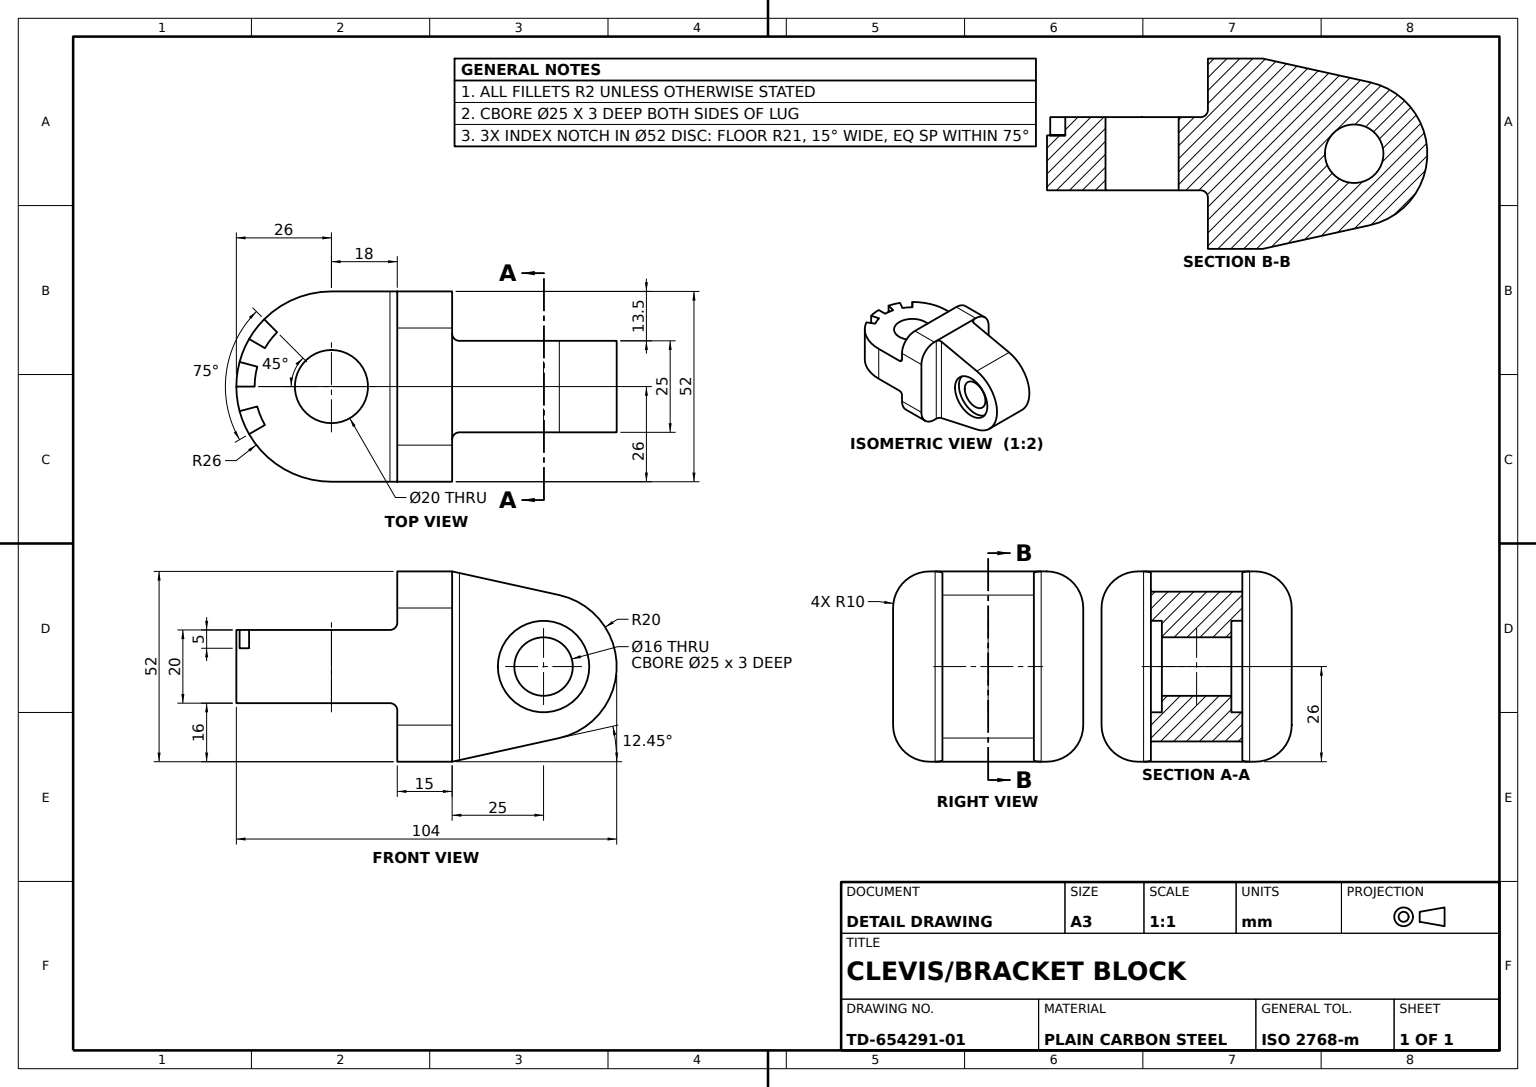
ISO-10303-21;
HEADER;
FILE_DESCRIPTION((''),'2;1');
FILE_NAME('','',(''),(''),'','','');
FILE_SCHEMA(('AUTOMOTIVE_DESIGN'));
ENDSEC;
DATA;
#1=APPLICATION_CONTEXT('');
#2=PRODUCT_CONTEXT('',#1,'mechanical');
#3=PRODUCT('','','',(#2));
#4=PRODUCT_DEFINITION_FORMATION('','',#3);
#5=PRODUCT_DEFINITION_CONTEXT('',#1,'design');
#6=PRODUCT_DEFINITION('','',#4,#5);
#7=PRODUCT_DEFINITION_SHAPE('','',#6);
#8=(LENGTH_UNIT()NAMED_UNIT(*)SI_UNIT(.MILLI.,.METRE.));
#9=(NAMED_UNIT(*)PLANE_ANGLE_UNIT()SI_UNIT($,.RADIAN.));
#10=(NAMED_UNIT(*)SI_UNIT($,.STERADIAN.)SOLID_ANGLE_UNIT());
#11=UNCERTAINTY_MEASURE_WITH_UNIT(LENGTH_MEASURE(1.E-05),#8,'distance_accuracy_value','');
#12=(GEOMETRIC_REPRESENTATION_CONTEXT(3)GLOBAL_UNCERTAINTY_ASSIGNED_CONTEXT((#11))GLOBAL_UNIT_ASSIGNED_CONTEXT((#8,#9,#10))REPRESENTATION_CONTEXT('',''));
#13=CARTESIAN_POINT('',(-25.5,-10.,-10.));
#14=VERTEX_POINT('',#13);
#15=CARTESIAN_POINT('',(-25.5,-10.,10.));
#16=VERTEX_POINT('',#15);
#17=CARTESIAN_POINT('',(-25.5,-10.,0.));
#18=DIRECTION('',(0.,1.,0.));
#19=DIRECTION('',(0.,0.,1.));
#20=AXIS2_PLACEMENT_3D('',#17,#18,#19);
#21=CIRCLE('',#20,10.);
#22=EDGE_CURVE('',#14,#16,#21,.T.);
#23=ORIENTED_EDGE('',*,*,#22,.T.);
#24=EDGE_CURVE('',#16,#14,#21,.T.);
#25=ORIENTED_EDGE('',*,*,#24,.T.);
#26=EDGE_LOOP('',(#23,#25));
#27=FACE_BOUND('',#26,.T.);
#28=CARTESIAN_POINT('',(-25.5,-10.,26.));
#29=VERTEX_POINT('',#28);
#30=CARTESIAN_POINT('',(-9.5,-10.,26.));
#31=VERTEX_POINT('',#30);
#32=CARTESIAN_POINT('',(0.,-10.,26.));
#33=DIRECTION('',(1.,0.,0.));
#34=VECTOR('',#33,1000.);
#35=LINE('',#32,#34);
#36=EDGE_CURVE('',#29,#31,#35,.T.);
#37=ORIENTED_EDGE('',*,*,#36,.F.);
#38=CARTESIAN_POINT('',(-25.5,-10.,-26.));
#39=VERTEX_POINT('',#38);
#40=DIRECTION('',(0.,-1.,0.));
#41=AXIS2_PLACEMENT_3D('',#17,#40,#19);
#42=CIRCLE('',#41,26.);
#43=EDGE_CURVE('',#29,#39,#42,.T.);
#44=ORIENTED_EDGE('',*,*,#43,.T.);
#45=CARTESIAN_POINT('',(-9.5,-10.,-26.));
#46=VERTEX_POINT('',#45);
#47=CARTESIAN_POINT('',(0.,-10.,-26.));
#48=LINE('',#47,#34);
#49=EDGE_CURVE('',#39,#46,#48,.T.);
#50=ORIENTED_EDGE('',*,*,#49,.T.);
#51=VECTOR('',#19,1000.);
#52=LINE('',#30,#51);
#53=EDGE_CURVE('',#46,#31,#52,.T.);
#54=ORIENTED_EDGE('',*,*,#53,.T.);
#55=EDGE_LOOP('',(#37,#44,#50,#54));
#56=FACE_OUTER_BOUND('',#55,.T.);
#57=CARTESIAN_POINT('',(0.,-10.,0.));
#58=AXIS2_PLACEMENT_3D('',#57,#18,#19);
#59=PLANE('',#58);
#60=ADVANCED_FACE('',(#27,#56),#59,.F.);
#61=CARTESIAN_POINT('',(24.5,0.,9.5));
#62=VERTEX_POINT('',#61);
#63=CARTESIAN_POINT('',(24.5,0.,-9.5));
#64=VERTEX_POINT('',#63);
#65=CARTESIAN_POINT('',(24.5,0.,-12.5));
#66=DIRECTION('',(0.,0.,-1.));
#67=VECTOR('',#66,1000.);
#68=LINE('',#65,#67);
#69=EDGE_CURVE('',#62,#64,#68,.T.);
#70=ORIENTED_EDGE('',*,*,#69,.F.);
#71=CARTESIAN_POINT('',(40.5,0.,9.5));
#72=VERTEX_POINT('',#71);
#73=CARTESIAN_POINT('',(32.5,0.,9.5));
#74=AXIS2_PLACEMENT_3D('',#73,#19,#33);
#75=CIRCLE('',#74,8.);
#76=EDGE_CURVE('',#62,#72,#75,.T.);
#77=ORIENTED_EDGE('',*,*,#76,.T.);
#78=CARTESIAN_POINT('',(40.5,0.,-9.5));
#79=VERTEX_POINT('',#78);
#80=CARTESIAN_POINT('',(40.5,0.,-12.5));
#81=LINE('',#80,#67);
#82=EDGE_CURVE('',#72,#79,#81,.T.);
#83=ORIENTED_EDGE('',*,*,#82,.T.);
#84=CARTESIAN_POINT('',(32.5,0.,-9.5));
#85=DIRECTION('',(-1.,0.,0.));
#86=AXIS2_PLACEMENT_3D('',#84,#66,#85);
#87=CIRCLE('',#86,8.);
#88=EDGE_CURVE('',#79,#64,#87,.T.);
#89=ORIENTED_EDGE('',*,*,#88,.T.);
#90=EDGE_LOOP('',(#70,#77,#83,#89));
#91=FACE_OUTER_BOUND('',#90,.T.);
#92=CARTESIAN_POINT('',(32.5,0.,-12.5));
#93=AXIS2_PLACEMENT_3D('',#92,#66,#85);
#94=CYLINDRICAL_SURFACE('',#93,8.);
#95=ADVANCED_FACE('',(#91),#94,.F.);
#96=EDGE_CURVE('',#64,#79,#87,.T.);
#97=ORIENTED_EDGE('',*,*,#96,.F.);
#98=ORIENTED_EDGE('',*,*,#88,.F.);
#99=EDGE_LOOP('',(#97,#98));
#100=FACE_BOUND('',#99,.T.);
#101=CARTESIAN_POINT('',(20.,0.,-9.5));
#102=VERTEX_POINT('',#101);
#103=CARTESIAN_POINT('',(45.,0.,-9.5));
#104=VERTEX_POINT('',#103);
#105=CIRCLE('',#86,12.5);
#106=EDGE_CURVE('',#102,#104,#105,.T.);
#107=ORIENTED_EDGE('',*,*,#106,.T.);
#108=EDGE_CURVE('',#104,#102,#105,.T.);
#109=ORIENTED_EDGE('',*,*,#108,.T.);
#110=EDGE_LOOP('',(#107,#109));
#111=FACE_OUTER_BOUND('',#110,.T.);
#112=AXIS2_PLACEMENT_3D('',#78,#19,#33);
#113=PLANE('',#112);
#114=ADVANCED_FACE('',(#100,#111),#113,.F.);
#115=CARTESIAN_POINT('',(-40.349242,5.,-14.849242));
#116=VERTEX_POINT('',#115);
#117=CARTESIAN_POINT('',(-43.686533,5.,-10.5));
#118=VERTEX_POINT('',#117);
#119=CARTESIAN_POINT('',(-25.5,5.,0.));
#120=AXIS2_PLACEMENT_3D('',#119,#18,#19);
#121=CIRCLE('',#120,21.);
#122=EDGE_CURVE('',#116,#118,#121,.T.);
#123=ORIENTED_EDGE('',*,*,#122,.F.);
#124=CARTESIAN_POINT('',(-43.884776,5.,-18.384776));
#125=VERTEX_POINT('',#124);
#126=CARTESIAN_POINT('',(-12.75,5.,12.75));
#127=DIRECTION('',(0.707106781,0.,0.707106781));
#128=VECTOR('',#127,1000.);
#129=LINE('',#126,#128);
#130=EDGE_CURVE('',#125,#116,#129,.T.);
#131=ORIENTED_EDGE('',*,*,#130,.F.);
#132=CARTESIAN_POINT('',(-48.01666,5.,-13.));
#133=VERTEX_POINT('',#132);
#134=CIRCLE('',#120,26.);
#135=EDGE_CURVE('',#125,#133,#134,.T.);
#136=ORIENTED_EDGE('',*,*,#135,.T.);
#137=CARTESIAN_POINT('',(-6.375,5.,11.041824));
#138=DIRECTION('',(-0.866025404,0.,-0.5));
#139=VECTOR('',#138,1000.);
#140=LINE('',#137,#139);
#141=EDGE_CURVE('',#118,#133,#140,.T.);
#142=ORIENTED_EDGE('',*,*,#141,.F.);
#143=EDGE_LOOP('',(#123,#131,#136,#142));
#144=FACE_OUTER_BOUND('',#143,.T.);
#145=CARTESIAN_POINT('',(0.,5.,0.));
#146=AXIS2_PLACEMENT_3D('',#145,#18,#19);
#147=PLANE('',#146);
#148=ADVANCED_FACE('',(#144),#147,.T.);
#149=CARTESIAN_POINT('',(-46.5,5.,0.));
#150=VERTEX_POINT('',#149);
#151=CARTESIAN_POINT('',(-46.5,10.,0.));
#152=VERTEX_POINT('',#151);
#153=VECTOR('',#18,1000.);
#154=LINE('',#149,#153);
#155=EDGE_CURVE('',#150,#152,#154,.T.);
#156=ORIENTED_EDGE('',*,*,#155,.T.);
#157=CARTESIAN_POINT('',(-45.784442,10.,-5.4352));
#158=VERTEX_POINT('',#157);
#159=CARTESIAN_POINT('',(-25.5,10.,0.));
#160=AXIS2_PLACEMENT_3D('',#159,#18,#19);
#161=CIRCLE('',#160,21.);
#162=EDGE_CURVE('',#158,#152,#161,.T.);
#163=ORIENTED_EDGE('',*,*,#162,.F.);
#164=CARTESIAN_POINT('',(-45.784442,5.,-5.4352));
#165=VERTEX_POINT('',#164);
#166=LINE('',#164,#153);
#167=EDGE_CURVE('',#165,#158,#166,.T.);
#168=ORIENTED_EDGE('',*,*,#167,.F.);
#169=EDGE_CURVE('',#165,#150,#121,.T.);
#170=ORIENTED_EDGE('',*,*,#169,.T.);
#171=EDGE_LOOP('',(#156,#163,#168,#170));
#172=FACE_OUTER_BOUND('',#171,.T.);
#173=CYLINDRICAL_SURFACE('',#120,21.);
#174=ADVANCED_FACE('',(#172),#173,.T.);
#175=ORIENTED_EDGE('',*,*,#36,.T.);
#176=CARTESIAN_POINT('',(-7.5,-12.,26.));
#177=VERTEX_POINT('',#176);
#178=CARTESIAN_POINT('',(-9.5,-12.,26.));
#179=AXIS2_PLACEMENT_3D('',#178,#66,#85);
#180=CIRCLE('',#179,2.);
#181=EDGE_CURVE('',#31,#177,#180,.T.);
#182=ORIENTED_EDGE('',*,*,#181,.T.);
#183=CARTESIAN_POINT('',(-7.5,-16.,26.));
#184=VERTEX_POINT('',#183);
#185=VECTOR('',#40,1000.);
#186=LINE('',#183,#185);
#187=EDGE_CURVE('',#177,#184,#186,.T.);
#188=ORIENTED_EDGE('',*,*,#187,.T.);
#189=CARTESIAN_POINT('',(7.5,-16.,26.));
#190=VERTEX_POINT('',#189);
#191=VECTOR('',#85,1000.);
#192=LINE('',#189,#191);
#193=EDGE_CURVE('',#190,#184,#192,.T.);
#194=ORIENTED_EDGE('',*,*,#193,.F.);
#195=CARTESIAN_POINT('',(7.5,16.,26.));
#196=VERTEX_POINT('',#195);
#197=LINE('',#189,#185);
#198=EDGE_CURVE('',#196,#190,#197,.T.);
#199=ORIENTED_EDGE('',*,*,#198,.F.);
#200=CARTESIAN_POINT('',(-7.5,16.,26.));
#201=VERTEX_POINT('',#200);
#202=LINE('',#195,#191);
#203=EDGE_CURVE('',#196,#201,#202,.T.);
#204=ORIENTED_EDGE('',*,*,#203,.T.);
#205=CARTESIAN_POINT('',(-7.5,12.,26.));
#206=VERTEX_POINT('',#205);
#207=EDGE_CURVE('',#201,#206,#186,.T.);
#208=ORIENTED_EDGE('',*,*,#207,.T.);
#209=CARTESIAN_POINT('',(-9.5,10.,26.));
#210=VERTEX_POINT('',#209);
#211=CARTESIAN_POINT('',(-9.5,12.,26.));
#212=AXIS2_PLACEMENT_3D('',#211,#66,#85);
#213=CIRCLE('',#212,2.);
#214=EDGE_CURVE('',#206,#210,#213,.T.);
#215=ORIENTED_EDGE('',*,*,#214,.T.);
#216=CARTESIAN_POINT('',(-25.5,10.,26.));
#217=VERTEX_POINT('',#216);
#218=CARTESIAN_POINT('',(0.,10.,26.));
#219=LINE('',#218,#34);
#220=EDGE_CURVE('',#217,#210,#219,.T.);
#221=ORIENTED_EDGE('',*,*,#220,.F.);
#222=LINE('',#216,#185);
#223=EDGE_CURVE('',#217,#29,#222,.T.);
#224=ORIENTED_EDGE('',*,*,#223,.T.);
#225=EDGE_LOOP('',(#175,#182,#188,#194,#199,#204,#208,#215,#221,#224));
#226=FACE_OUTER_BOUND('',#225,.T.);
#227=AXIS2_PLACEMENT_3D('',#189,#66,#85);
#228=PLANE('',#227);
#229=ADVANCED_FACE('',(#226),#228,.F.);
#230=CARTESIAN_POINT('',(9.5,25.558518,12.5));
#231=VERTEX_POINT('',#230);
#232=CARTESIAN_POINT('',(9.5,-25.558518,12.5));
#233=VERTEX_POINT('',#232);
#234=CARTESIAN_POINT('',(9.5,-26.,12.5));
#235=LINE('',#234,#185);
#236=EDGE_CURVE('',#231,#233,#235,.T.);
#237=ORIENTED_EDGE('',*,*,#236,.F.);
#238=CARTESIAN_POINT('',(7.5,26.,14.5));
#239=VERTEX_POINT('',#238);
#240=CARTESIAN_POINT('',(7.5,26.,13.328427));
#241=CARTESIAN_POINT('',(8.328427,25.817132,12.5));
#242=(BOUNDED_CURVE()B_SPLINE_CURVE(3,(#238,#240,#241,#230),.UNSPECIFIED.,.F.,.F.)B_SPLINE_CURVE_WITH_KNOTS((4,4),(0.,1.570796327),.UNSPECIFIED.)CURVE()GEOMETRIC_REPRESENTATION_ITEM()RATIONAL_B_SPLINE_CURVE((1.,0.804737854,0.804737854,1.))REPRESENTATION_ITEM(''));
#243=EDGE_CURVE('',#239,#231,#242,.T.);
#244=ORIENTED_EDGE('',*,*,#243,.F.);
#245=CARTESIAN_POINT('',(7.5,-26.,14.5));
#246=VERTEX_POINT('',#245);
#247=LINE('',#238,#153);
#248=EDGE_CURVE('',#246,#239,#247,.T.);
#249=ORIENTED_EDGE('',*,*,#248,.F.);
#250=CARTESIAN_POINT('',(8.328427,-25.817132,12.5));
#251=CARTESIAN_POINT('',(7.5,-26.,13.328427));
#252=(BOUNDED_CURVE()B_SPLINE_CURVE(3,(#232,#250,#251,#245),.UNSPECIFIED.,.F.,.F.)B_SPLINE_CURVE_WITH_KNOTS((4,4),(1.570796327,3.141592654),.UNSPECIFIED.)CURVE()GEOMETRIC_REPRESENTATION_ITEM()RATIONAL_B_SPLINE_CURVE((1.,0.804737854,0.804737854,1.))REPRESENTATION_ITEM(''));
#253=EDGE_CURVE('',#233,#246,#252,.T.);
#254=ORIENTED_EDGE('',*,*,#253,.F.);
#255=EDGE_LOOP('',(#237,#244,#249,#254));
#256=FACE_OUTER_BOUND('',#255,.T.);
#257=CARTESIAN_POINT('',(9.5,0.,14.5));
#258=AXIS2_PLACEMENT_3D('',#257,#18,#19);
#259=CYLINDRICAL_SURFACE('',#258,2.);
#260=ADVANCED_FACE('',(#256),#259,.F.);
#261=CARTESIAN_POINT('',(7.5,-26.,-14.5));
#262=VERTEX_POINT('',#261);
#263=CARTESIAN_POINT('',(7.5,-26.,12.5));
#264=LINE('',#263,#67);
#265=EDGE_CURVE('',#246,#262,#264,.T.);
#266=ORIENTED_EDGE('',*,*,#265,.T.);
#267=CARTESIAN_POINT('',(9.5,-25.558518,-12.5));
#268=VERTEX_POINT('',#267);
#269=CARTESIAN_POINT('',(7.5,-26.,-13.328427));
#270=CARTESIAN_POINT('',(8.328427,-25.817132,-12.5));
#271=(BOUNDED_CURVE()B_SPLINE_CURVE(3,(#261,#269,#270,#267),.UNSPECIFIED.,.F.,.F.)B_SPLINE_CURVE_WITH_KNOTS((4,4),(0.,1.570796327),.UNSPECIFIED.)CURVE()GEOMETRIC_REPRESENTATION_ITEM()RATIONAL_B_SPLINE_CURVE((1.,0.804737854,0.804737854,1.))REPRESENTATION_ITEM(''));
#272=EDGE_CURVE('',#262,#268,#271,.T.);
#273=ORIENTED_EDGE('',*,*,#272,.T.);
#274=CARTESIAN_POINT('',(36.811041,-19.529847,-12.5));
#275=VERTEX_POINT('',#274);
#276=CARTESIAN_POINT('',(7.5,-26.,-12.5));
#277=DIRECTION('',(0.976492353,0.215552047,0.));
#278=VECTOR('',#277,1000.);
#279=LINE('',#276,#278);
#280=EDGE_CURVE('',#268,#275,#279,.T.);
#281=ORIENTED_EDGE('',*,*,#280,.T.);
#282=CARTESIAN_POINT('',(36.811041,-19.529847,12.5));
#283=VERTEX_POINT('',#282);
#284=LINE('',#282,#67);
#285=EDGE_CURVE('',#283,#275,#284,.T.);
#286=ORIENTED_EDGE('',*,*,#285,.F.);
#287=LINE('',#263,#278);
#288=EDGE_CURVE('',#233,#283,#287,.T.);
#289=ORIENTED_EDGE('',*,*,#288,.F.);
#290=ORIENTED_EDGE('',*,*,#253,.T.);
#291=EDGE_LOOP('',(#266,#273,#281,#286,#289,#290));
#292=FACE_OUTER_BOUND('',#291,.T.);
#293=DIRECTION('',(-0.215552047,0.976492353,0.));
#294=DIRECTION('',(-0.976492353,-0.215552047,0.));
#295=AXIS2_PLACEMENT_3D('',#263,#293,#294);
#296=PLANE('',#295);
#297=ADVANCED_FACE('',(#292),#296,.F.);
#298=CARTESIAN_POINT('',(-43.686533,5.,10.5));
#299=VERTEX_POINT('',#298);
#300=CARTESIAN_POINT('',(-48.01666,5.,13.));
#301=VERTEX_POINT('',#300);
#302=CARTESIAN_POINT('',(-6.375,5.,-11.041824));
#303=DIRECTION('',(-0.866025404,0.,0.5));
#304=VECTOR('',#303,1000.);
#305=LINE('',#302,#304);
#306=EDGE_CURVE('',#299,#301,#305,.T.);
#307=ORIENTED_EDGE('',*,*,#306,.F.);
#308=CARTESIAN_POINT('',(-45.784442,5.,5.4352));
#309=VERTEX_POINT('',#308);
#310=EDGE_CURVE('',#309,#299,#121,.T.);
#311=ORIENTED_EDGE('',*,*,#310,.F.);
#312=CARTESIAN_POINT('',(-50.614071,5.,6.729295));
#313=VERTEX_POINT('',#312);
#314=CARTESIAN_POINT('',(-1.708176,5.,-6.375));
#315=DIRECTION('',(0.965925826,0.,-0.258819045));
#316=VECTOR('',#315,1000.);
#317=LINE('',#314,#316);
#318=EDGE_CURVE('',#313,#309,#317,.T.);
#319=ORIENTED_EDGE('',*,*,#318,.F.);
#320=EDGE_CURVE('',#313,#301,#134,.T.);
#321=ORIENTED_EDGE('',*,*,#320,.T.);
#322=EDGE_LOOP('',(#307,#311,#319,#321));
#323=FACE_OUTER_BOUND('',#322,.T.);
#324=ADVANCED_FACE('',(#323),#147,.T.);
#325=CARTESIAN_POINT('',(-7.5,-12.,-26.));
#326=VERTEX_POINT('',#325);
#327=LINE('',#325,#67);
#328=EDGE_CURVE('',#177,#326,#327,.T.);
#329=ORIENTED_EDGE('',*,*,#328,.F.);
#330=ORIENTED_EDGE('',*,*,#181,.F.);
#331=ORIENTED_EDGE('',*,*,#53,.F.);
#332=CARTESIAN_POINT('',(-9.5,-12.,-26.));
#333=AXIS2_PLACEMENT_3D('',#332,#19,#33);
#334=CIRCLE('',#333,2.);
#335=EDGE_CURVE('',#326,#46,#334,.T.);
#336=ORIENTED_EDGE('',*,*,#335,.F.);
#337=EDGE_LOOP('',(#329,#330,#331,#336));
#338=FACE_OUTER_BOUND('',#337,.T.);
#339=CARTESIAN_POINT('',(-9.5,-12.,16.));
#340=AXIS2_PLACEMENT_3D('',#339,#19,#33);
#341=CYLINDRICAL_SURFACE('',#340,2.);
#342=ADVANCED_FACE('',(#338),#341,.F.);
#343=ORIENTED_EDGE('',*,*,#167,.T.);
#344=CARTESIAN_POINT('',(-50.614071,10.,-6.729295));
#345=VERTEX_POINT('',#344);
#346=CARTESIAN_POINT('',(-1.708176,10.,6.375));
#347=DIRECTION('',(0.965925826,0.,0.258819045));
#348=VECTOR('',#347,1000.);
#349=LINE('',#346,#348);
#350=EDGE_CURVE('',#345,#158,#349,.T.);
#351=ORIENTED_EDGE('',*,*,#350,.F.);
#352=CARTESIAN_POINT('',(-50.614071,5.,-6.729295));
#353=VERTEX_POINT('',#352);
#354=LINE('',#352,#153);
#355=EDGE_CURVE('',#353,#345,#354,.T.);
#356=ORIENTED_EDGE('',*,*,#355,.F.);
#357=CARTESIAN_POINT('',(-1.708176,5.,6.375));
#358=LINE('',#357,#348);
#359=EDGE_CURVE('',#353,#165,#358,.T.);
#360=ORIENTED_EDGE('',*,*,#359,.T.);
#361=EDGE_LOOP('',(#343,#351,#356,#360));
#362=FACE_OUTER_BOUND('',#361,.T.);
#363=DIRECTION('',(-0.258819045,0.,0.965925826));
#364=AXIS2_PLACEMENT_3D('',#357,#363,#347);
#365=PLANE('',#364);
#366=ADVANCED_FACE('',(#362),#365,.T.);
#367=CARTESIAN_POINT('',(20.,0.,9.5));
#368=VERTEX_POINT('',#367);
#369=CARTESIAN_POINT('',(45.,0.,9.5));
#370=VERTEX_POINT('',#369);
#371=CIRCLE('',#74,12.5);
#372=EDGE_CURVE('',#368,#370,#371,.T.);
#373=ORIENTED_EDGE('',*,*,#372,.T.);
#374=EDGE_CURVE('',#370,#368,#371,.T.);
#375=ORIENTED_EDGE('',*,*,#374,.T.);
#376=EDGE_LOOP('',(#373,#375));
#377=FACE_OUTER_BOUND('',#376,.T.);
#378=EDGE_CURVE('',#72,#62,#75,.T.);
#379=ORIENTED_EDGE('',*,*,#378,.F.);
#380=ORIENTED_EDGE('',*,*,#76,.F.);
#381=EDGE_LOOP('',(#379,#380));
#382=FACE_BOUND('',#381,.T.);
#383=AXIS2_PLACEMENT_3D('',#71,#66,#85);
#384=PLANE('',#383);
#385=ADVANCED_FACE('',(#377,#382),#384,.F.);
#386=CARTESIAN_POINT('',(45.,0.,12.5));
#387=VERTEX_POINT('',#386);
#388=LINE('',#386,#51);
#389=EDGE_CURVE('',#370,#387,#388,.T.);
#390=ORIENTED_EDGE('',*,*,#389,.T.);
#391=CARTESIAN_POINT('',(20.,0.,12.5));
#392=VERTEX_POINT('',#391);
#393=CARTESIAN_POINT('',(32.5,0.,12.5));
#394=AXIS2_PLACEMENT_3D('',#393,#19,#33);
#395=CIRCLE('',#394,12.5);
#396=EDGE_CURVE('',#387,#392,#395,.T.);
#397=ORIENTED_EDGE('',*,*,#396,.T.);
#398=LINE('',#391,#51);
#399=EDGE_CURVE('',#368,#392,#398,.T.);
#400=ORIENTED_EDGE('',*,*,#399,.F.);
#401=ORIENTED_EDGE('',*,*,#374,.F.);
#402=EDGE_LOOP('',(#390,#397,#400,#401));
#403=FACE_OUTER_BOUND('',#402,.T.);
#404=CYLINDRICAL_SURFACE('',#394,12.5);
#405=ADVANCED_FACE('',(#403),#404,.F.);
#406=ORIENTED_EDGE('',*,*,#187,.F.);
#407=ORIENTED_EDGE('',*,*,#328,.T.);
#408=CARTESIAN_POINT('',(-7.5,-16.,-26.));
#409=VERTEX_POINT('',#408);
#410=LINE('',#408,#153);
#411=EDGE_CURVE('',#409,#326,#410,.T.);
#412=ORIENTED_EDGE('',*,*,#411,.F.);
#413=CARTESIAN_POINT('',(-7.5,-26.,-16.));
#414=VERTEX_POINT('',#413);
#415=CARTESIAN_POINT('',(-7.5,-16.,-16.));
#416=AXIS2_PLACEMENT_3D('',#415,#33,#66);
#417=CIRCLE('',#416,10.);
#418=EDGE_CURVE('',#414,#409,#417,.T.);
#419=ORIENTED_EDGE('',*,*,#418,.F.);
#420=CARTESIAN_POINT('',(-7.5,-26.,16.));
#421=VERTEX_POINT('',#420);
#422=LINE('',#420,#67);
#423=EDGE_CURVE('',#421,#414,#422,.T.);
#424=ORIENTED_EDGE('',*,*,#423,.F.);
#425=CARTESIAN_POINT('',(-7.5,-16.,16.));
#426=AXIS2_PLACEMENT_3D('',#425,#33,#66);
#427=CIRCLE('',#426,10.);
#428=EDGE_CURVE('',#184,#421,#427,.T.);
#429=ORIENTED_EDGE('',*,*,#428,.F.);
#430=EDGE_LOOP('',(#406,#407,#412,#419,#424,#429));
#431=FACE_OUTER_BOUND('',#430,.T.);
#432=PLANE('',#426);
#433=ADVANCED_FACE('',(#431),#432,.F.);
#434=ORIENTED_EDGE('',*,*,#135,.F.);
#435=CARTESIAN_POINT('',(-43.884776,10.,-18.384776));
#436=VERTEX_POINT('',#435);
#437=LINE('',#124,#153);
#438=EDGE_CURVE('',#125,#436,#437,.T.);
#439=ORIENTED_EDGE('',*,*,#438,.T.);
#440=CARTESIAN_POINT('',(-25.5,10.,-26.));
#441=VERTEX_POINT('',#440);
#442=AXIS2_PLACEMENT_3D('',#159,#40,#19);
#443=CIRCLE('',#442,26.);
#444=EDGE_CURVE('',#436,#441,#443,.T.);
#445=ORIENTED_EDGE('',*,*,#444,.T.);
#446=LINE('',#440,#185);
#447=EDGE_CURVE('',#441,#39,#446,.T.);
#448=ORIENTED_EDGE('',*,*,#447,.T.);
#449=ORIENTED_EDGE('',*,*,#43,.F.);
#450=ORIENTED_EDGE('',*,*,#223,.F.);
#451=CARTESIAN_POINT('',(-48.01666,10.,13.));
#452=VERTEX_POINT('',#451);
#453=EDGE_CURVE('',#217,#452,#443,.T.);
#454=ORIENTED_EDGE('',*,*,#453,.T.);
#455=LINE('',#300,#153);
#456=EDGE_CURVE('',#301,#452,#455,.T.);
#457=ORIENTED_EDGE('',*,*,#456,.F.);
#458=ORIENTED_EDGE('',*,*,#320,.F.);
#459=CARTESIAN_POINT('',(-50.614071,10.,6.729295));
#460=VERTEX_POINT('',#459);
#461=LINE('',#312,#153);
#462=EDGE_CURVE('',#313,#460,#461,.T.);
#463=ORIENTED_EDGE('',*,*,#462,.T.);
#464=CARTESIAN_POINT('',(-51.5,10.,0.));
#465=VERTEX_POINT('',#464);
#466=EDGE_CURVE('',#460,#465,#443,.T.);
#467=ORIENTED_EDGE('',*,*,#466,.T.);
#468=CARTESIAN_POINT('',(-51.5,5.,0.));
#469=VERTEX_POINT('',#468);
#470=LINE('',#468,#153);
#471=EDGE_CURVE('',#469,#465,#470,.T.);
#472=ORIENTED_EDGE('',*,*,#471,.F.);
#473=EDGE_CURVE('',#353,#469,#134,.T.);
#474=ORIENTED_EDGE('',*,*,#473,.F.);
#475=ORIENTED_EDGE('',*,*,#355,.T.);
#476=CARTESIAN_POINT('',(-48.01666,10.,-13.));
#477=VERTEX_POINT('',#476);
#478=EDGE_CURVE('',#345,#477,#443,.T.);
#479=ORIENTED_EDGE('',*,*,#478,.T.);
#480=LINE('',#132,#153);
#481=EDGE_CURVE('',#133,#477,#480,.T.);
#482=ORIENTED_EDGE('',*,*,#481,.F.);
#483=EDGE_LOOP('',(#434,#439,#445,#448,#449,#450,#454,#457,#458,#463,#467,#472,#474,#475,#479,#482));
#484=FACE_OUTER_BOUND('',#483,.T.);
#485=AXIS2_PLACEMENT_3D('',#159,#40,#66);
#486=CYLINDRICAL_SURFACE('',#485,26.);
#487=ADVANCED_FACE('',(#484),#486,.T.);
#488=CARTESIAN_POINT('',(-40.349242,10.,-14.849242));
#489=VERTEX_POINT('',#488);
#490=LINE('',#115,#153);
#491=EDGE_CURVE('',#116,#489,#490,.T.);
#492=ORIENTED_EDGE('',*,*,#491,.T.);
#493=CARTESIAN_POINT('',(-12.75,10.,12.75));
#494=LINE('',#493,#128);
#495=EDGE_CURVE('',#436,#489,#494,.T.);
#496=ORIENTED_EDGE('',*,*,#495,.F.);
#497=ORIENTED_EDGE('',*,*,#438,.F.);
#498=ORIENTED_EDGE('',*,*,#130,.T.);
#499=EDGE_LOOP('',(#492,#496,#497,#498));
#500=FACE_OUTER_BOUND('',#499,.T.);
#501=DIRECTION('',(-0.707106781,0.,0.707106781));
#502=AXIS2_PLACEMENT_3D('',#126,#501,#127);
#503=PLANE('',#502);
#504=ADVANCED_FACE('',(#500),#503,.T.);
#505=CARTESIAN_POINT('',(9.5,25.558518,-12.5));
#506=VERTEX_POINT('',#505);
#507=CARTESIAN_POINT('',(7.5,26.,-14.5));
#508=VERTEX_POINT('',#507);
#509=CARTESIAN_POINT('',(8.328427,25.817132,-12.5));
#510=CARTESIAN_POINT('',(7.5,26.,-13.328427));
#511=(BOUNDED_CURVE()B_SPLINE_CURVE(3,(#505,#509,#510,#507),.UNSPECIFIED.,.F.,.F.)B_SPLINE_CURVE_WITH_KNOTS((4,4),(1.570796327,3.141592654),.UNSPECIFIED.)CURVE()GEOMETRIC_REPRESENTATION_ITEM()RATIONAL_B_SPLINE_CURVE((1.,0.804737854,0.804737854,1.))REPRESENTATION_ITEM(''));
#512=EDGE_CURVE('',#506,#508,#511,.T.);
#513=ORIENTED_EDGE('',*,*,#512,.T.);
#514=CARTESIAN_POINT('',(7.5,26.,12.5));
#515=LINE('',#514,#67);
#516=EDGE_CURVE('',#239,#508,#515,.T.);
#517=ORIENTED_EDGE('',*,*,#516,.F.);
#518=ORIENTED_EDGE('',*,*,#243,.T.);
#519=CARTESIAN_POINT('',(36.811041,19.529847,12.5));
#520=VERTEX_POINT('',#519);
#521=DIRECTION('',(-0.976492353,0.215552047,0.));
#522=VECTOR('',#521,1000.);
#523=LINE('',#514,#522);
#524=EDGE_CURVE('',#520,#231,#523,.T.);
#525=ORIENTED_EDGE('',*,*,#524,.F.);
#526=CARTESIAN_POINT('',(36.811041,19.529847,-12.5));
#527=VERTEX_POINT('',#526);
#528=LINE('',#519,#67);
#529=EDGE_CURVE('',#520,#527,#528,.T.);
#530=ORIENTED_EDGE('',*,*,#529,.T.);
#531=CARTESIAN_POINT('',(7.5,26.,-12.5));
#532=LINE('',#531,#522);
#533=EDGE_CURVE('',#527,#506,#532,.T.);
#534=ORIENTED_EDGE('',*,*,#533,.T.);
#535=EDGE_LOOP('',(#513,#517,#518,#525,#530,#534));
#536=FACE_OUTER_BOUND('',#535,.T.);
#537=DIRECTION('',(-0.215552047,-0.976492353,0.));
#538=DIRECTION('',(0.976492353,-0.215552047,0.));
#539=AXIS2_PLACEMENT_3D('',#514,#537,#538);
#540=PLANE('',#539);
#541=ADVANCED_FACE('',(#536),#540,.F.);
#542=CARTESIAN_POINT('',(-7.5,12.,-26.));
#543=VERTEX_POINT('',#542);
#544=CARTESIAN_POINT('',(-7.5,12.,16.));
#545=LINE('',#544,#51);
#546=EDGE_CURVE('',#543,#206,#545,.T.);
#547=ORIENTED_EDGE('',*,*,#546,.T.);
#548=ORIENTED_EDGE('',*,*,#207,.F.);
#549=CARTESIAN_POINT('',(-7.5,26.,16.));
#550=VERTEX_POINT('',#549);
#551=CARTESIAN_POINT('',(-7.5,16.,16.));
#552=AXIS2_PLACEMENT_3D('',#551,#33,#19);
#553=CIRCLE('',#552,10.);
#554=EDGE_CURVE('',#550,#201,#553,.T.);
#555=ORIENTED_EDGE('',*,*,#554,.F.);
#556=CARTESIAN_POINT('',(-7.5,26.,-16.));
#557=VERTEX_POINT('',#556);
#558=LINE('',#549,#51);
#559=EDGE_CURVE('',#557,#550,#558,.T.);
#560=ORIENTED_EDGE('',*,*,#559,.F.);
#561=CARTESIAN_POINT('',(-7.5,16.,-26.));
#562=VERTEX_POINT('',#561);
#563=CARTESIAN_POINT('',(-7.5,16.,-16.));
#564=AXIS2_PLACEMENT_3D('',#563,#33,#19);
#565=CIRCLE('',#564,10.);
#566=EDGE_CURVE('',#562,#557,#565,.T.);
#567=ORIENTED_EDGE('',*,*,#566,.F.);
#568=EDGE_CURVE('',#543,#562,#410,.T.);
#569=ORIENTED_EDGE('',*,*,#568,.F.);
#570=EDGE_LOOP('',(#547,#548,#555,#560,#567,#569));
#571=FACE_OUTER_BOUND('',#570,.T.);
#572=ADVANCED_FACE('',(#571),#432,.F.);
#573=CARTESIAN_POINT('',(-25.5,10.,-10.));
#574=VERTEX_POINT('',#573);
#575=LINE('',#573,#185);
#576=EDGE_CURVE('',#574,#14,#575,.T.);
#577=ORIENTED_EDGE('',*,*,#576,.F.);
#578=CARTESIAN_POINT('',(-25.5,10.,10.));
#579=VERTEX_POINT('',#578);
#580=CIRCLE('',#160,10.);
#581=EDGE_CURVE('',#574,#579,#580,.T.);
#582=ORIENTED_EDGE('',*,*,#581,.T.);
#583=LINE('',#578,#185);
#584=EDGE_CURVE('',#579,#16,#583,.T.);
#585=ORIENTED_EDGE('',*,*,#584,.T.);
#586=ORIENTED_EDGE('',*,*,#22,.F.);
#587=EDGE_LOOP('',(#577,#582,#585,#586));
#588=FACE_OUTER_BOUND('',#587,.T.);
#589=CYLINDRICAL_SURFACE('',#485,10.);
#590=ADVANCED_FACE('',(#588),#589,.F.);
#591=CARTESIAN_POINT('',(0.,10.,0.));
#592=LINE('',#591,#34);
#593=EDGE_CURVE('',#465,#152,#592,.T.);
#594=ORIENTED_EDGE('',*,*,#593,.T.);
#595=ORIENTED_EDGE('',*,*,#155,.F.);
#596=LINE('',#145,#34);
#597=EDGE_CURVE('',#469,#150,#596,.T.);
#598=ORIENTED_EDGE('',*,*,#597,.F.);
#599=ORIENTED_EDGE('',*,*,#471,.T.);
#600=EDGE_LOOP('',(#594,#595,#598,#599));
#601=FACE_OUTER_BOUND('',#600,.T.);
#602=AXIS2_PLACEMENT_3D('',#145,#19,#33);
#603=PLANE('',#602);
#604=ADVANCED_FACE('',(#601),#603,.F.);
#605=CARTESIAN_POINT('',(7.5,-26.,16.));
#606=VERTEX_POINT('',#605);
#607=CARTESIAN_POINT('',(7.5,-16.,16.));
#608=AXIS2_PLACEMENT_3D('',#607,#33,#66);
#609=CIRCLE('',#608,10.);
#610=EDGE_CURVE('',#190,#606,#609,.T.);
#611=ORIENTED_EDGE('',*,*,#610,.F.);
#612=ORIENTED_EDGE('',*,*,#193,.T.);
#613=ORIENTED_EDGE('',*,*,#428,.T.);
#614=LINE('',#605,#191);
#615=EDGE_CURVE('',#606,#421,#614,.T.);
#616=ORIENTED_EDGE('',*,*,#615,.F.);
#617=EDGE_LOOP('',(#611,#612,#613,#616));
#618=FACE_OUTER_BOUND('',#617,.T.);
#619=AXIS2_PLACEMENT_3D('',#607,#85,#19);
#620=CYLINDRICAL_SURFACE('',#619,10.);
#621=ADVANCED_FACE('',(#618),#620,.T.);
#622=ORIENTED_EDGE('',*,*,#566,.T.);
#623=CARTESIAN_POINT('',(7.5,26.,-16.));
#624=VERTEX_POINT('',#623);
#625=LINE('',#623,#191);
#626=EDGE_CURVE('',#624,#557,#625,.T.);
#627=ORIENTED_EDGE('',*,*,#626,.F.);
#628=CARTESIAN_POINT('',(7.5,16.,-26.));
#629=VERTEX_POINT('',#628);
#630=CARTESIAN_POINT('',(7.5,16.,-16.));
#631=AXIS2_PLACEMENT_3D('',#630,#33,#19);
#632=CIRCLE('',#631,10.);
#633=EDGE_CURVE('',#629,#624,#632,.T.);
#634=ORIENTED_EDGE('',*,*,#633,.F.);
#635=LINE('',#628,#191);
#636=EDGE_CURVE('',#629,#562,#635,.T.);
#637=ORIENTED_EDGE('',*,*,#636,.T.);
#638=EDGE_LOOP('',(#622,#627,#634,#637));
#639=FACE_OUTER_BOUND('',#638,.T.);
#640=AXIS2_PLACEMENT_3D('',#630,#85,#19);
#641=CYLINDRICAL_SURFACE('',#640,10.);
#642=ADVANCED_FACE('',(#639),#641,.T.);
#643=CARTESIAN_POINT('',(7.5,-16.,-26.));
#644=VERTEX_POINT('',#643);
#645=LINE('',#643,#153);
#646=EDGE_CURVE('',#644,#629,#645,.T.);
#647=ORIENTED_EDGE('',*,*,#646,.F.);
#648=LINE('',#643,#191);
#649=EDGE_CURVE('',#644,#409,#648,.T.);
#650=ORIENTED_EDGE('',*,*,#649,.T.);
#651=ORIENTED_EDGE('',*,*,#411,.T.);
#652=ORIENTED_EDGE('',*,*,#335,.T.);
#653=ORIENTED_EDGE('',*,*,#49,.F.);
#654=ORIENTED_EDGE('',*,*,#447,.F.);
#655=CARTESIAN_POINT('',(-9.5,10.,-26.));
#656=VERTEX_POINT('',#655);
#657=CARTESIAN_POINT('',(0.,10.,-26.));
#658=LINE('',#657,#34);
#659=EDGE_CURVE('',#441,#656,#658,.T.);
#660=ORIENTED_EDGE('',*,*,#659,.T.);
#661=CARTESIAN_POINT('',(-9.5,12.,-26.));
#662=AXIS2_PLACEMENT_3D('',#661,#19,#33);
#663=CIRCLE('',#662,2.);
#664=EDGE_CURVE('',#656,#543,#663,.T.);
#665=ORIENTED_EDGE('',*,*,#664,.T.);
#666=ORIENTED_EDGE('',*,*,#568,.T.);
#667=ORIENTED_EDGE('',*,*,#636,.F.);
#668=EDGE_LOOP('',(#647,#650,#651,#652,#653,#654,#660,#665,#666,#667));
#669=FACE_OUTER_BOUND('',#668,.T.);
#670=AXIS2_PLACEMENT_3D('',#643,#19,#33);
#671=PLANE('',#670);
#672=ADVANCED_FACE('',(#669),#671,.F.);
#673=CARTESIAN_POINT('',(-43.686533,10.,-10.5));
#674=VERTEX_POINT('',#673);
#675=EDGE_CURVE('',#489,#674,#161,.T.);
#676=ORIENTED_EDGE('',*,*,#675,.F.);
#677=ORIENTED_EDGE('',*,*,#491,.F.);
#678=ORIENTED_EDGE('',*,*,#122,.T.);
#679=LINE('',#117,#153);
#680=EDGE_CURVE('',#118,#674,#679,.T.);
#681=ORIENTED_EDGE('',*,*,#680,.T.);
#682=EDGE_LOOP('',(#676,#677,#678,#681));
#683=FACE_OUTER_BOUND('',#682,.T.);
#684=ADVANCED_FACE('',(#683),#173,.T.);
#685=CARTESIAN_POINT('',(-43.686533,10.,10.5));
#686=VERTEX_POINT('',#685);
#687=CARTESIAN_POINT('',(-6.375,10.,-11.041824));
#688=LINE('',#687,#304);
#689=EDGE_CURVE('',#686,#452,#688,.T.);
#690=ORIENTED_EDGE('',*,*,#689,.F.);
#691=LINE('',#298,#153);
#692=EDGE_CURVE('',#299,#686,#691,.T.);
#693=ORIENTED_EDGE('',*,*,#692,.F.);
#694=ORIENTED_EDGE('',*,*,#306,.T.);
#695=ORIENTED_EDGE('',*,*,#456,.T.);
#696=EDGE_LOOP('',(#690,#693,#694,#695));
#697=FACE_OUTER_BOUND('',#696,.T.);
#698=DIRECTION('',(-0.5,0.,-0.866025404));
#699=AXIS2_PLACEMENT_3D('',#302,#698,#303);
#700=PLANE('',#699);
#701=ADVANCED_FACE('',(#697),#700,.T.);
#702=ORIENTED_EDGE('',*,*,#236,.T.);
#703=ORIENTED_EDGE('',*,*,#288,.T.);
#704=CIRCLE('',#394,20.);
#705=EDGE_CURVE('',#283,#520,#704,.T.);
#706=ORIENTED_EDGE('',*,*,#705,.T.);
#707=ORIENTED_EDGE('',*,*,#524,.T.);
#708=EDGE_LOOP('',(#702,#703,#706,#707));
#709=FACE_OUTER_BOUND('',#708,.T.);
#710=EDGE_CURVE('',#392,#387,#395,.T.);
#711=ORIENTED_EDGE('',*,*,#710,.F.);
#712=ORIENTED_EDGE('',*,*,#396,.F.);
#713=EDGE_LOOP('',(#711,#712));
#714=FACE_BOUND('',#713,.T.);
#715=PLANE('',#394);
#716=ADVANCED_FACE('',(#709,#714),#715,.T.);
#717=ORIENTED_EDGE('',*,*,#359,.F.);
#718=ORIENTED_EDGE('',*,*,#473,.T.);
#719=ORIENTED_EDGE('',*,*,#597,.T.);
#720=ORIENTED_EDGE('',*,*,#169,.F.);
#721=EDGE_LOOP('',(#717,#718,#719,#720));
#722=FACE_OUTER_BOUND('',#721,.T.);
#723=ADVANCED_FACE('',(#722),#147,.T.);
#724=ORIENTED_EDGE('',*,*,#162,.T.);
#725=ORIENTED_EDGE('',*,*,#593,.F.);
#726=ORIENTED_EDGE('',*,*,#466,.F.);
#727=CARTESIAN_POINT('',(-45.784442,10.,5.4352));
#728=VERTEX_POINT('',#727);
#729=CARTESIAN_POINT('',(-1.708176,10.,-6.375));
#730=LINE('',#729,#316);
#731=EDGE_CURVE('',#460,#728,#730,.T.);
#732=ORIENTED_EDGE('',*,*,#731,.T.);
#733=EDGE_CURVE('',#728,#686,#161,.T.);
#734=ORIENTED_EDGE('',*,*,#733,.T.);
#735=ORIENTED_EDGE('',*,*,#689,.T.);
#736=ORIENTED_EDGE('',*,*,#453,.F.);
#737=ORIENTED_EDGE('',*,*,#220,.T.);
#738=CARTESIAN_POINT('',(-9.5,10.,0.));
#739=LINE('',#738,#67);
#740=EDGE_CURVE('',#210,#656,#739,.T.);
#741=ORIENTED_EDGE('',*,*,#740,.T.);
#742=ORIENTED_EDGE('',*,*,#659,.F.);
#743=ORIENTED_EDGE('',*,*,#444,.F.);
#744=ORIENTED_EDGE('',*,*,#495,.T.);
#745=ORIENTED_EDGE('',*,*,#675,.T.);
#746=CARTESIAN_POINT('',(-6.375,10.,11.041824));
#747=LINE('',#746,#139);
#748=EDGE_CURVE('',#674,#477,#747,.T.);
#749=ORIENTED_EDGE('',*,*,#748,.T.);
#750=ORIENTED_EDGE('',*,*,#478,.F.);
#751=ORIENTED_EDGE('',*,*,#350,.T.);
#752=EDGE_LOOP('',(#724,#725,#726,#732,#734,#735,#736,#737,#741,#742,#743,#744,#745,#749,#750,#751));
#753=FACE_OUTER_BOUND('',#752,.T.);
#754=EDGE_CURVE('',#579,#574,#580,.T.);
#755=ORIENTED_EDGE('',*,*,#754,.F.);
#756=ORIENTED_EDGE('',*,*,#581,.F.);
#757=EDGE_LOOP('',(#755,#756));
#758=FACE_BOUND('',#757,.T.);
#759=AXIS2_PLACEMENT_3D('',#591,#18,#19);
#760=PLANE('',#759);
#761=ADVANCED_FACE('',(#753,#758),#760,.T.);
#762=CARTESIAN_POINT('',(20.,0.,-12.5));
#763=VERTEX_POINT('',#762);
#764=CARTESIAN_POINT('',(45.,0.,-12.5));
#765=VERTEX_POINT('',#764);
#766=CIRCLE('',#93,12.5);
#767=EDGE_CURVE('',#763,#765,#766,.T.);
#768=ORIENTED_EDGE('',*,*,#767,.T.);
#769=LINE('',#764,#67);
#770=EDGE_CURVE('',#104,#765,#769,.T.);
#771=ORIENTED_EDGE('',*,*,#770,.F.);
#772=ORIENTED_EDGE('',*,*,#106,.F.);
#773=LINE('',#762,#67);
#774=EDGE_CURVE('',#102,#763,#773,.T.);
#775=ORIENTED_EDGE('',*,*,#774,.T.);
#776=EDGE_LOOP('',(#768,#771,#772,#775));
#777=FACE_OUTER_BOUND('',#776,.T.);
#778=CYLINDRICAL_SURFACE('',#93,12.5);
#779=ADVANCED_FACE('',(#777),#778,.F.);
#780=ORIENTED_EDGE('',*,*,#529,.F.);
#781=ORIENTED_EDGE('',*,*,#705,.F.);
#782=ORIENTED_EDGE('',*,*,#285,.T.);
#783=AXIS2_PLACEMENT_3D('',#92,#19,#33);
#784=CIRCLE('',#783,20.);
#785=EDGE_CURVE('',#275,#527,#784,.T.);
#786=ORIENTED_EDGE('',*,*,#785,.T.);
#787=EDGE_LOOP('',(#780,#781,#782,#786));
#788=FACE_OUTER_BOUND('',#787,.T.);
#789=AXIS2_PLACEMENT_3D('',#393,#66,#85);
#790=CYLINDRICAL_SURFACE('',#789,20.);
#791=ADVANCED_FACE('',(#788),#790,.T.);
#792=CARTESIAN_POINT('',(9.5,0.,-12.5));
#793=LINE('',#792,#153);
#794=EDGE_CURVE('',#268,#506,#793,.T.);
#795=ORIENTED_EDGE('',*,*,#794,.F.);
#796=ORIENTED_EDGE('',*,*,#272,.F.);
#797=CARTESIAN_POINT('',(7.5,-16.,-14.5));
#798=LINE('',#797,#185);
#799=EDGE_CURVE('',#508,#262,#798,.T.);
#800=ORIENTED_EDGE('',*,*,#799,.F.);
#801=ORIENTED_EDGE('',*,*,#512,.F.);
#802=EDGE_LOOP('',(#795,#796,#800,#801));
#803=FACE_OUTER_BOUND('',#802,.T.);
#804=CARTESIAN_POINT('',(9.5,-16.,-14.5));
#805=AXIS2_PLACEMENT_3D('',#804,#40,#66);
#806=CYLINDRICAL_SURFACE('',#805,2.);
#807=ADVANCED_FACE('',(#803),#806,.F.);
#808=ORIENTED_EDGE('',*,*,#141,.T.);
#809=ORIENTED_EDGE('',*,*,#481,.T.);
#810=ORIENTED_EDGE('',*,*,#748,.F.);
#811=ORIENTED_EDGE('',*,*,#680,.F.);
#812=EDGE_LOOP('',(#808,#809,#810,#811));
#813=FACE_OUTER_BOUND('',#812,.T.);
#814=DIRECTION('',(0.5,0.,-0.866025404));
#815=AXIS2_PLACEMENT_3D('',#137,#814,#138);
#816=PLANE('',#815);
#817=ADVANCED_FACE('',(#813),#816,.T.);
#818=ORIENTED_EDGE('',*,*,#559,.T.);
#819=CARTESIAN_POINT('',(7.5,26.,16.));
#820=VERTEX_POINT('',#819);
#821=LINE('',#819,#191);
#822=EDGE_CURVE('',#820,#550,#821,.T.);
#823=ORIENTED_EDGE('',*,*,#822,.F.);
#824=LINE('',#819,#51);
#825=EDGE_CURVE('',#239,#820,#824,.T.);
#826=ORIENTED_EDGE('',*,*,#825,.F.);
#827=ORIENTED_EDGE('',*,*,#516,.T.);
#828=EDGE_CURVE('',#624,#508,#824,.T.);
#829=ORIENTED_EDGE('',*,*,#828,.F.);
#830=ORIENTED_EDGE('',*,*,#626,.T.);
#831=EDGE_LOOP('',(#818,#823,#826,#827,#829,#830));
#832=FACE_OUTER_BOUND('',#831,.T.);
#833=AXIS2_PLACEMENT_3D('',#819,#40,#66);
#834=PLANE('',#833);
#835=ADVANCED_FACE('',(#832),#834,.F.);
#836=ORIENTED_EDGE('',*,*,#399,.T.);
#837=ORIENTED_EDGE('',*,*,#710,.T.);
#838=ORIENTED_EDGE('',*,*,#389,.F.);
#839=ORIENTED_EDGE('',*,*,#372,.F.);
#840=EDGE_LOOP('',(#836,#837,#838,#839));
#841=FACE_OUTER_BOUND('',#840,.T.);
#842=ADVANCED_FACE('',(#841),#404,.F.);
#843=ORIENTED_EDGE('',*,*,#546,.F.);
#844=ORIENTED_EDGE('',*,*,#664,.F.);
#845=ORIENTED_EDGE('',*,*,#740,.F.);
#846=ORIENTED_EDGE('',*,*,#214,.F.);
#847=EDGE_LOOP('',(#843,#844,#845,#846));
#848=FACE_OUTER_BOUND('',#847,.T.);
#849=CARTESIAN_POINT('',(-9.5,12.,0.));
#850=AXIS2_PLACEMENT_3D('',#849,#66,#85);
#851=CYLINDRICAL_SURFACE('',#850,2.);
#852=ADVANCED_FACE('',(#848),#851,.F.);
#853=EDGE_CURVE('',#765,#763,#766,.T.);
#854=ORIENTED_EDGE('',*,*,#853,.F.);
#855=ORIENTED_EDGE('',*,*,#767,.F.);
#856=EDGE_LOOP('',(#854,#855));
#857=FACE_BOUND('',#856,.T.);
#858=ORIENTED_EDGE('',*,*,#785,.F.);
#859=ORIENTED_EDGE('',*,*,#280,.F.);
#860=ORIENTED_EDGE('',*,*,#794,.T.);
#861=ORIENTED_EDGE('',*,*,#533,.F.);
#862=EDGE_LOOP('',(#858,#859,#860,#861));
#863=FACE_OUTER_BOUND('',#862,.T.);
#864=PLANE('',#783);
#865=ADVANCED_FACE('',(#857,#863),#864,.F.);
#866=ORIENTED_EDGE('',*,*,#615,.T.);
#867=ORIENTED_EDGE('',*,*,#423,.T.);
#868=CARTESIAN_POINT('',(7.5,-26.,-16.));
#869=VERTEX_POINT('',#868);
#870=LINE('',#868,#191);
#871=EDGE_CURVE('',#869,#414,#870,.T.);
#872=ORIENTED_EDGE('',*,*,#871,.F.);
#873=LINE('',#605,#67);
#874=EDGE_CURVE('',#262,#869,#873,.T.);
#875=ORIENTED_EDGE('',*,*,#874,.F.);
#876=ORIENTED_EDGE('',*,*,#265,.F.);
#877=EDGE_CURVE('',#606,#246,#873,.T.);
#878=ORIENTED_EDGE('',*,*,#877,.F.);
#879=EDGE_LOOP('',(#866,#867,#872,#875,#876,#878));
#880=FACE_OUTER_BOUND('',#879,.T.);
#881=AXIS2_PLACEMENT_3D('',#605,#18,#19);
#882=PLANE('',#881);
#883=ADVANCED_FACE('',(#880),#882,.F.);
#884=ORIENTED_EDGE('',*,*,#692,.T.);
#885=ORIENTED_EDGE('',*,*,#733,.F.);
#886=LINE('',#308,#153);
#887=EDGE_CURVE('',#309,#728,#886,.T.);
#888=ORIENTED_EDGE('',*,*,#887,.F.);
#889=ORIENTED_EDGE('',*,*,#310,.T.);
#890=EDGE_LOOP('',(#884,#885,#888,#889));
#891=FACE_OUTER_BOUND('',#890,.T.);
#892=ADVANCED_FACE('',(#891),#173,.T.);
#893=ORIENTED_EDGE('',*,*,#649,.F.);
#894=CARTESIAN_POINT('',(7.5,-16.,-16.));
#895=AXIS2_PLACEMENT_3D('',#894,#33,#66);
#896=CIRCLE('',#895,10.);
#897=EDGE_CURVE('',#869,#644,#896,.T.);
#898=ORIENTED_EDGE('',*,*,#897,.F.);
#899=ORIENTED_EDGE('',*,*,#871,.T.);
#900=ORIENTED_EDGE('',*,*,#418,.T.);
#901=EDGE_LOOP('',(#893,#898,#899,#900));
#902=FACE_OUTER_BOUND('',#901,.T.);
#903=AXIS2_PLACEMENT_3D('',#894,#85,#19);
#904=CYLINDRICAL_SURFACE('',#903,10.);
#905=ADVANCED_FACE('',(#902),#904,.T.);
#906=ORIENTED_EDGE('',*,*,#897,.T.);
#907=ORIENTED_EDGE('',*,*,#646,.T.);
#908=ORIENTED_EDGE('',*,*,#633,.T.);
#909=ORIENTED_EDGE('',*,*,#828,.T.);
#910=ORIENTED_EDGE('',*,*,#799,.T.);
#911=ORIENTED_EDGE('',*,*,#874,.T.);
#912=EDGE_LOOP('',(#906,#907,#908,#909,#910,#911));
#913=FACE_OUTER_BOUND('',#912,.T.);
#914=PLANE('',#608);
#915=ADVANCED_FACE('',(#913),#914,.T.);
#916=ORIENTED_EDGE('',*,*,#576,.T.);
#917=ORIENTED_EDGE('',*,*,#24,.F.);
#918=ORIENTED_EDGE('',*,*,#584,.F.);
#919=ORIENTED_EDGE('',*,*,#754,.T.);
#920=EDGE_LOOP('',(#916,#917,#918,#919));
#921=FACE_OUTER_BOUND('',#920,.T.);
#922=ADVANCED_FACE('',(#921),#589,.F.);
#923=CARTESIAN_POINT('',(7.5,16.,16.));
#924=AXIS2_PLACEMENT_3D('',#923,#33,#19);
#925=CIRCLE('',#924,10.);
#926=EDGE_CURVE('',#820,#196,#925,.T.);
#927=ORIENTED_EDGE('',*,*,#926,.F.);
#928=ORIENTED_EDGE('',*,*,#822,.T.);
#929=ORIENTED_EDGE('',*,*,#554,.T.);
#930=ORIENTED_EDGE('',*,*,#203,.F.);
#931=EDGE_LOOP('',(#927,#928,#929,#930));
#932=FACE_OUTER_BOUND('',#931,.T.);
#933=AXIS2_PLACEMENT_3D('',#923,#85,#19);
#934=CYLINDRICAL_SURFACE('',#933,10.);
#935=ADVANCED_FACE('',(#932),#934,.T.);
#936=ORIENTED_EDGE('',*,*,#462,.F.);
#937=ORIENTED_EDGE('',*,*,#318,.T.);
#938=ORIENTED_EDGE('',*,*,#887,.T.);
#939=ORIENTED_EDGE('',*,*,#731,.F.);
#940=EDGE_LOOP('',(#936,#937,#938,#939));
#941=FACE_OUTER_BOUND('',#940,.T.);
#942=DIRECTION('',(0.258819045,0.,0.965925826));
#943=AXIS2_PLACEMENT_3D('',#314,#942,#315);
#944=PLANE('',#943);
#945=ADVANCED_FACE('',(#941),#944,.T.);
#946=ORIENTED_EDGE('',*,*,#69,.T.);
#947=ORIENTED_EDGE('',*,*,#96,.T.);
#948=ORIENTED_EDGE('',*,*,#82,.F.);
#949=ORIENTED_EDGE('',*,*,#378,.T.);
#950=EDGE_LOOP('',(#946,#947,#948,#949));
#951=FACE_OUTER_BOUND('',#950,.T.);
#952=ADVANCED_FACE('',(#951),#94,.F.);
#953=ORIENTED_EDGE('',*,*,#108,.F.);
#954=ORIENTED_EDGE('',*,*,#770,.T.);
#955=ORIENTED_EDGE('',*,*,#853,.T.);
#956=ORIENTED_EDGE('',*,*,#774,.F.);
#957=EDGE_LOOP('',(#953,#954,#955,#956));
#958=FACE_OUTER_BOUND('',#957,.T.);
#959=ADVANCED_FACE('',(#958),#778,.F.);
#960=ORIENTED_EDGE('',*,*,#825,.T.);
#961=ORIENTED_EDGE('',*,*,#926,.T.);
#962=ORIENTED_EDGE('',*,*,#198,.T.);
#963=ORIENTED_EDGE('',*,*,#610,.T.);
#964=ORIENTED_EDGE('',*,*,#877,.T.);
#965=ORIENTED_EDGE('',*,*,#248,.T.);
#966=EDGE_LOOP('',(#960,#961,#962,#963,#964,#965));
#967=FACE_OUTER_BOUND('',#966,.T.);
#968=ADVANCED_FACE('',(#967),#914,.T.);
#969=CLOSED_SHELL('',(#60,#95,#114,#148,#174,#229,#260,#297,#324,#342,#366,#385,#405,#433,#487,#504,#541,#572,#590,#604,#621,#642,#672,#684,#701,#716,#723,#761,#779,#791,#807,#817,#835,#842,#852,#865,#883,#892,#905,#915,#922,#935,#945,#952,#959,#968));
#970=MANIFOLD_SOLID_BREP('',#969);
#971=ADVANCED_BREP_SHAPE_REPRESENTATION('',(#970),#12);
#972=SHAPE_DEFINITION_REPRESENTATION(#7,#971);
ENDSEC;
END-ISO-10303-21;
